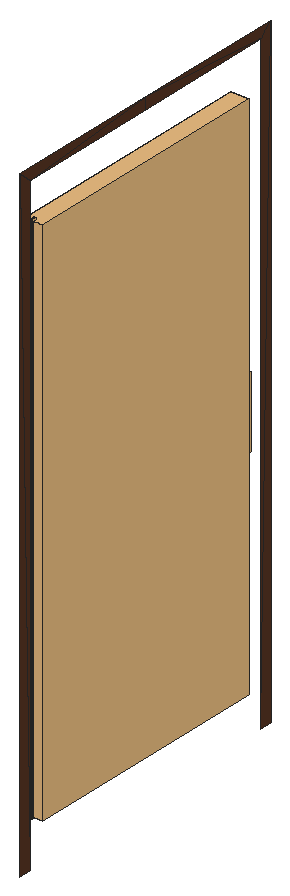
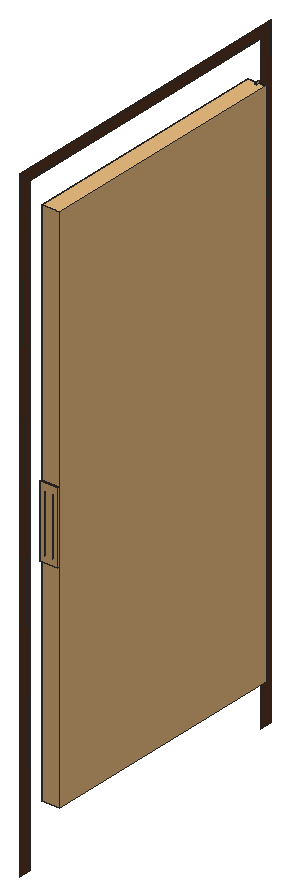
# SketchUp Ruby script. Lengths in inches.
U = 1.inch
M = Sketchup.active_model
def pt(a) = Geom::Point3d.new(a.map { |v| v * U })
def face(e, loops, mat)
  f = e.add_face(loops[0].map { |a| pt(a) })
  loops[1..].each { |l| e.add_face(l.map { |a| pt(a) }).erase! }
  f.material = f.back_material = mat if mat
  f
end
# faces: each face lists its corners as indices into pts; further lists are holes
def faces(e, pts, list, mat = nil) = list.each { |f| face(e, (f[0].is_a?(Array) ? f : [f]).map { |l| l.map { |i| pts[i] } }, mat) }
# xy, xz, yz: faces in a plane at the given z, y or x. An outline is a flat list of corners, or four numbers for a rectangle; further outlines are holes
def ring(l) = l.size == 4 ? [[l[0], l[1]], [l[2], l[1]], [l[2], l[3]], [l[0], l[3]]] : l.each_slice(2).to_a
def flat(e, list, mat, &to3) = list.each { |f| face(e, (f[0].is_a?(Array) ? f : [f]).map { |l| ring(l).map { |u, v| to3.(u, v) } }, mat) }
def xy(e, z, list, mat = nil) = flat(e, list, mat) { |x, y| [x, y, z] }
def xz(e, y, list, mat = nil) = flat(e, list, mat) { |x, z| [x, y, z] }
def yz(e, x, list, mat = nil) = flat(e, list, mat) { |y, z| [x, y, z] }
def lines(e, pts, list) = list.each { |a, b| e.add_line(pt(pts[a]), pt(pts[b])) }
# prism: a flat outline (further loops are holes) pulled along v
def prism(e, loops, v, mat = nil)
  f = face(e, loops, mat); d = Geom::Vector3d.new(v.map { |x| x * U })
  f.pushpull(f.normal.samedirection?(d) ? d.length : -d.length)
end
def box(e, o, s, mat = nil) = prism(e, [[o, [o[0] + s[0], o[1], o[2]], [o[0] + s[0], o[1] + s[1], o[2]], [o[0], o[1] + s[1], o[2]]]], [0, 0, s[2]], mat)
def at(x, y, z, deg = 0) = Geom::Transformation.translation(pt([x, y, z])) * Geom::Transformation.rotation(ORIGIN, Z_AXIS, deg.degrees)
def axes(o, x, y, z) = Geom::Transformation.new([*x, 0, *y, 0, *z, 0, *pt(o).to_a, 1])
def part(name) = M.definitions.add(name)
# library, detail: a bought-in or finely detailed component or shape, given as its bounding box
def library(name, o, s) = part(name).tap { |d| box(d.entities, o, s) }
def detail(e, o, s) = box(e.add_group.entities, o, s)
def put(e, d, t, mat = nil) = e.add_instance(d, t).tap { |i| i.material = mat if mat }
def group(e, t, mat = nil) = e.add_group.tap { |g| g.transformation = t; g.material = mat if mat }.entities
root = M.entities
M.materials.add("Material \#0").color = [86, 53, 35]
M.materials.add("Material \#1").color = [140, 140, 140]
c1 = library("3DGeom~9_Defintion",[456.52,-471.89,-18.89],[5.57,1000,5.49])
c2 = library("3DGeom~7_Defintion",[455.56,-471.94,-18.85],[5.55,1000,5.48])
c3 = part("3DGeom~8_Defintion")
xz(c3.entities,-471.94,[[458.125,-17.29,459.53,-16.11,457.73,-17.15],[458.125,-17.29,458.54,-17.29,459.53,-16.11],[458.54,-17.29,458.93,-17.15,459.53,-16.11],[457.73,-17.15,459.53,-16.11,457.42,-16.88],[458.93,-17.15,459.25,-16.88,459.53,-16.11],
  [457.42,-16.88,459.53,-16.11,457.21,-16.52],[459.25,-16.88,459.46,-16.52,459.53,-16.11],[457.21,-16.52,459.53,-16.11,457.14,-16.11],[457.14,-16.11,459.53,-16.11,457.21,-15.7],[459.53,-16.11,457.42,-15.34,457.21,-15.7],
  [459.53,-16.11,457.73,-15.07,457.42,-15.34],[459.53,-16.11,458.125,-14.93,457.73,-15.07],[459.53,-16.11,458.54,-14.93,458.125,-14.93],[459.53,-16.11,458.93,-15.07,458.54,-14.93],[459.53,-16.11,459.25,-15.34,458.93,-15.07],
  [459.53,-16.11,459.46,-15.7,459.25,-15.34]],"Material \#1")
xz(c3.entities,-416.39,[[458.125,-17.29,457.73,-17.15,459.53,-16.11],[458.125,-17.29,459.53,-16.11,458.54,-17.29],[458.54,-17.29,459.53,-16.11,458.93,-17.15],[457.73,-17.15,457.42,-16.88,459.53,-16.11],[458.93,-17.15,459.53,-16.11,459.25,-16.88],
  [457.42,-16.88,457.21,-16.52,459.53,-16.11],[459.25,-16.88,459.53,-16.11,459.46,-16.52],[457.21,-16.52,457.14,-16.11,459.53,-16.11],[457.14,-16.11,457.21,-15.7,459.53,-16.11],[459.53,-16.11,457.21,-15.7,457.42,-15.34],
  [459.53,-16.11,457.42,-15.34,457.73,-15.07],[459.53,-16.11,457.73,-15.07,458.125,-14.93],[459.53,-16.11,458.125,-14.93,458.54,-14.93],[459.53,-16.11,458.54,-14.93,458.93,-15.07],[459.53,-16.11,458.93,-15.07,459.25,-15.34],
  [459.53,-16.11,459.25,-15.34,459.46,-15.7]],"Material \#1")
xz(c3.entities,-27.5,[[458.125,-17.29,459.53,-16.11,457.73,-17.15],[458.125,-17.29,458.54,-17.29,459.53,-16.11],[458.54,-17.29,458.93,-17.15,459.53,-16.11],[457.73,-17.15,459.53,-16.11,457.42,-16.88],[458.93,-17.15,459.25,-16.88,459.53,-16.11],
  [457.42,-16.88,459.53,-16.11,457.21,-16.52],[459.25,-16.88,459.46,-16.52,459.53,-16.11],[457.21,-16.52,459.53,-16.11,457.14,-16.11],[457.14,-16.11,459.53,-16.11,457.21,-15.7],[459.53,-16.11,457.42,-15.34,457.21,-15.7],
  [459.53,-16.11,457.73,-15.07,457.42,-15.34],[459.53,-16.11,458.125,-14.93,457.73,-15.07],[459.53,-16.11,458.54,-14.93,458.125,-14.93],[459.53,-16.11,458.93,-15.07,458.54,-14.93],[459.53,-16.11,459.25,-15.34,458.93,-15.07],
  [459.53,-16.11,459.46,-15.7,459.25,-15.34]],"Material \#1")
xz(c3.entities,28.06,[[458.125,-17.29,457.73,-17.15,459.53,-16.11],[458.125,-17.29,459.53,-16.11,458.54,-17.29],[458.54,-17.29,459.53,-16.11,458.93,-17.15],[457.73,-17.15,457.42,-16.88,459.53,-16.11],[458.93,-17.15,459.53,-16.11,459.25,-16.88],
  [457.42,-16.88,457.21,-16.52,459.53,-16.11],[459.25,-16.88,459.53,-16.11,459.46,-16.52],[457.21,-16.52,457.14,-16.11,459.53,-16.11],[457.14,-16.11,457.21,-15.7,459.53,-16.11],[459.53,-16.11,457.21,-15.7,457.42,-15.34],
  [459.53,-16.11,457.42,-15.34,457.73,-15.07],[459.53,-16.11,457.73,-15.07,458.125,-14.93],[459.53,-16.11,458.125,-14.93,458.54,-14.93],[459.53,-16.11,458.54,-14.93,458.93,-15.07],[459.53,-16.11,458.93,-15.07,459.25,-15.34],
  [459.53,-16.11,459.25,-15.34,459.46,-15.7]],"Material \#1")
xz(c3.entities,472.5,[[458.125,-17.29,459.53,-16.11,457.73,-17.15],[458.125,-17.29,458.54,-17.29,459.53,-16.11],[458.54,-17.29,458.93,-17.15,459.53,-16.11],[457.73,-17.15,459.53,-16.11,457.42,-16.88],[458.93,-17.15,459.25,-16.88,459.53,-16.11],
  [457.42,-16.88,459.53,-16.11,457.21,-16.52],[459.25,-16.88,459.46,-16.52,459.53,-16.11],[457.21,-16.52,459.53,-16.11,457.14,-16.11],[457.14,-16.11,459.53,-16.11,457.21,-15.7],[459.53,-16.11,457.42,-15.34,457.21,-15.7],
  [459.53,-16.11,457.73,-15.07,457.42,-15.34],[459.53,-16.11,458.125,-14.93,457.73,-15.07],[459.53,-16.11,458.54,-14.93,458.125,-14.93],[459.53,-16.11,458.93,-15.07,458.54,-14.93],[459.53,-16.11,459.25,-15.34,458.93,-15.07],
  [459.53,-16.11,459.46,-15.7,459.25,-15.34]],"Material \#1")
xz(c3.entities,528.06,[[458.125,-17.29,457.73,-17.15,459.53,-16.11],[458.125,-17.29,459.53,-16.11,458.54,-17.29],[458.54,-17.29,459.53,-16.11,458.93,-17.15],[457.73,-17.15,457.42,-16.88,459.53,-16.11],[458.93,-17.15,459.53,-16.11,459.25,-16.88],
  [457.42,-16.88,457.21,-16.52,459.53,-16.11],[459.25,-16.88,459.53,-16.11,459.46,-16.52],[457.21,-16.52,457.14,-16.11,459.53,-16.11],[457.14,-16.11,457.21,-15.7,459.53,-16.11],[459.53,-16.11,457.21,-15.7,457.42,-15.34],
  [459.53,-16.11,457.42,-15.34,457.73,-15.07],[459.53,-16.11,457.73,-15.07,458.125,-14.93],[459.53,-16.11,458.125,-14.93,458.54,-14.93],[459.53,-16.11,458.54,-14.93,458.93,-15.07],[459.53,-16.11,458.93,-15.07,459.25,-15.34],
  [459.53,-16.11,459.25,-15.34,459.46,-15.7]],"Material \#1")
c4 = part("3DGeom~21_Defintion")
xy(c4.entities,73.08,[[-976.3,-241.71,23.7,-241.71,-976.3,-223.46],[23.7,-241.71,5.45,-223.46,-976.3,-223.46],[23.7,-241.71,23.7,0,5.45,-223.46],[5.45,-223.46,23.7,0,5.45,0],[23.7,0,23.7,241.71,5.45,223.46],
  [5.45,0,23.7,0,5.45,223.46],[-976.3,223.46,23.7,241.71,-976.3,241.71],[-976.3,223.46,5.45,223.46,23.7,241.71]],"Material \#0")
c5 = library("3DGeom~6_Defintion",[-5.59,-471.8,-48.03],[468.87,1000,73.72])
c6 = library("3DGeom~3_Defintion",[-83.33,-500,-350],[620.1,1000,533.33])
c7 = library("3DGeom~4_Defintion",[-18.02,-499.97,-221.16],[36.04,1000,262.12])
c8 = part("3DGeom~5_Defintion")
xy(c8.entities,-225.24,[[-0.79,-499.98,-2.33,-499.64,7.45,-496.14],[-0.79,-499.98,7.45,-496.14,1.58,-499.88],[1.58,-499.88,7.45,-496.14,3.84,-499.16],[-2.33,-499.64,7.4,-485.75,7.45,-496.14],[3.84,-499.16,7.45,-496.14,5.85,-497.89],
  [7.45,-496.14,7.4,-485.75,8.24,-487.08],[7.45,-496.14,8.24,-487.08,8.96,-489.34],[7.45,-496.14,8.96,-489.34,9.0625,-491.71],[7.45,-496.14,9.0625,-491.71,8.55,-494.03],[-7.4,-496.08,-8.24,-494.76,2.32,-482.2],
  [-8.24,-494.76,-8.96,-492.5,2.32,-482.2],[-8.96,-492.5,-9.0625,-490.125,2.32,-482.2],[-9.0625,-490.125,-8.55,-487.81,2.32,-482.2],[-8.55,-487.81,-7.45,-485.7,2.32,-482.2],[-7.45,-485.7,-5.85,-483.95,2.32,-482.2],
  [-5.85,-483.95,-3.84,-482.68,2.32,-482.2],[-3.84,-482.68,-1.58,-481.96,2.32,-482.2],[2.32,-482.2,-1.58,-481.96,0.79,-481.86],[0,481.82,-2.35,482.13,-6.92,496.71],[0,481.82,-6.92,496.71,1.55,482.04],
  [-2.35,482.13,-4.55,483.04,-6.92,496.71],[-4.55,483.04,-6.43,484.49,-6.92,496.71],[-6.43,484.49,-7.88,486.37,-6.92,496.71],[6.92,485.12,-1.55,499.8125,7.88,495.47],[6.92,485.12,7.88,495.47,7.88,486.37],
  [-7.88,486.37,-8.79,488.57,-6.92,496.71],[7.88,486.37,7.88,495.47,8.79,488.57],[-8.79,488.57,-9.1,490.92,-6.92,496.71],[8.79,488.57,7.88,495.47,9.1,490.92],[-9.1,490.92,-8.79,493.28,-6.92,496.71],
  [9.1,490.92,7.88,495.47,8.79,493.28],[-8.79,493.28,-7.88,495.47,-6.92,496.71],[7.88,495.47,-1.55,499.8125,0,500.02],[7.88,495.47,0,500.02,2.35,499.71],[7.88,495.47,2.35,499.71,4.55,498.8],
  [7.88,495.47,4.55,498.8,6.43,497.35]],"Material \#1")
xy(c8.entities,-221.57,[[-2.33,-499.64,-5.22,-498.37,7.4,-485.75],[-5.22,-498.37,-7.4,-496.08,5.22,-483.47],[-5.22,-498.37,5.22,-483.47,7.4,-485.75],[-7.4,-496.08,2.32,-482.2,5.22,-483.47],[1.55,482.04,-6.92,496.71,-4.55,498.8],
  [1.55,482.04,-4.55,498.8,4.55,483.04],[4.55,483.04,-4.55,498.8,-1.55,499.8125],[4.55,483.04,-1.55,499.8125,6.92,485.12]],"Material \#1")
xy(c8.entities,38.05,[[-2.33,-499.64,7.4,-485.75,-5.22,-498.37],[-5.22,-498.37,5.22,-483.47,-7.4,-496.08],[-5.22,-498.37,7.4,-485.75,5.22,-483.47],[-7.4,-496.08,5.22,-483.47,2.32,-482.2],[1.55,482.04,-4.55,498.8,-6.92,496.71],
  [1.55,482.04,4.55,483.04,-4.55,498.8],[4.55,483.04,-1.55,499.8125,-4.55,498.8],[4.55,483.04,6.92,485.12,-1.55,499.8125]],"Material \#1")
xy(c8.entities,41.72,[[-0.79,-499.98,7.45,-496.14,-2.33,-499.64],[-0.79,-499.98,1.58,-499.88,7.45,-496.14],[1.58,-499.88,3.84,-499.16,7.45,-496.14],[-2.33,-499.64,7.45,-496.14,7.4,-485.75],[3.84,-499.16,5.85,-497.89,7.45,-496.14],
  [7.45,-496.14,8.24,-487.08,7.4,-485.75],[7.45,-496.14,8.55,-494.03,9.0625,-491.71],[7.45,-496.14,8.96,-489.34,8.24,-487.08],[7.45,-496.14,9.0625,-491.71,8.96,-489.34],[-7.4,-496.08,2.32,-482.2,-8.24,-494.76],
  [-8.24,-494.76,2.32,-482.2,-8.96,-492.5],[-8.96,-492.5,2.32,-482.2,-9.0625,-490.125],[-9.0625,-490.125,2.32,-482.2,-8.55,-487.81],[-8.55,-487.81,2.32,-482.2,-7.45,-485.7],[-7.45,-485.7,2.32,-482.2,-5.85,-483.95],
  [-5.85,-483.95,2.32,-482.2,-3.84,-482.68],[-3.84,-482.68,2.32,-482.2,-1.58,-481.96],[2.32,-482.2,0.79,-481.86,-1.58,-481.96],[0,481.82,-6.92,496.71,-2.35,482.13],[0,481.82,1.55,482.04,-6.92,496.71],
  [-2.35,482.13,-6.92,496.71,-4.55,483.04],[-4.55,483.04,-6.92,496.71,-6.43,484.49],[-6.43,484.49,-6.92,496.71,-7.88,486.37],[6.92,485.12,7.88,495.47,-1.55,499.8125],[6.92,485.12,7.88,486.37,7.88,495.47],
  [-7.88,486.37,-6.92,496.71,-8.79,488.57],[7.88,486.37,8.79,488.57,7.88,495.47],[-8.79,488.57,-6.92,496.71,-9.1,490.92],[8.79,488.57,9.1,490.92,7.88,495.47],[-9.1,490.92,-6.92,496.71,-8.79,493.28],
  [9.1,490.92,8.79,493.28,7.88,495.47],[-8.79,493.28,-6.92,496.71,-7.88,495.47],[7.88,495.47,0,500.02,-1.55,499.8125],[7.88,495.47,2.35,499.71,0,500.02],[7.88,495.47,4.55,498.8,2.35,499.71],
  [7.88,495.47,6.43,497.35,4.55,498.8]],"Material \#1")
xy(root,7.66,[[363.16,355.99,363.12,356,363.12,356.03],[363.16,355.99,363.12,356.03,363.16,356.01],[363.16,355.99,363.16,356.01,363.2,356],[363.12,356,363.08,356.05,363.09,356.07],[363.12,356,363.09,356.07,363.12,356.03],
  [363.2,356,363.16,356.01,363.19,356.03],[363.2,356,363.19,356.03,363.23,356.05],[363.19,356.03,363.22,356.07,363.23,356.05],[363.08,356.05,363.06,356.12,363.07,356.13],[363.08,356.05,363.07,356.13,363.09,356.07],
  [363.23,356.05,363.22,356.07,363.26,356.12],[363.22,356.07,363.25,356.13,363.26,356.12],[363.06,356.12,363.04,356.2,363.06,356.2],[363.06,356.12,363.06,356.2,363.07,356.13],[363.26,356.12,363.25,356.13,363.27,356.2],
  [363.25,356.13,363.26,356.2,363.27,356.2],[363.04,356.2,363.04,356.29,363.06,356.28],[363.04,356.2,363.06,356.28,363.06,356.2],[363.26,356.2,363.26,356.28,363.27,356.29],[363.26,356.2,363.27,356.29,363.27,356.2],
  [363.06,356.28,363.04,356.29,363.07,356.36],[363.26,356.28,363.25,356.36,363.26,356.37],[363.26,356.28,363.26,356.37,363.27,356.29],[363.04,356.29,363.06,356.37,363.07,356.36],[363.07,356.36,363.06,356.37,363.09,356.42],
  [363.25,356.36,363.22,356.42,363.23,356.4375],[363.25,356.36,363.23,356.4375,363.26,356.37],[363.06,356.37,363.08,356.4375,363.09,356.42],[363.09,356.42,363.08,356.4375,363.12,356.46],[363.22,356.42,363.19,356.46,363.2,356.48],
  [363.22,356.42,363.2,356.48,363.23,356.4375],[363.08,356.4375,363.12,356.48,363.12,356.46],[363.12,356.46,363.12,356.48,363.16,356.47],[363.19,356.46,363.16,356.47,363.16,356.49],[363.19,356.46,363.16,356.49,363.2,356.48],
  [363.16,356.47,363.12,356.48,363.16,356.49]],"Material \#1")
xy(root,7.68,[[363.16,355.99,363.16,356.01,363.12,356],[363.16,355.99,363.19,356.03,363.16,356.01],[363.16,355.99,363.2,356,363.19,356.03],[363.12,356,363.12,356.03,363.08,356.05],[363.12,356,363.16,356.01,363.12,356.03],
  [363.2,356,363.22,356.07,363.19,356.03],[363.2,356,363.23,356.05,363.22,356.07],[363.12,356.03,363.09,356.07,363.08,356.05],[363.08,356.05,363.09,356.07,363.06,356.12],[363.23,356.05,363.25,356.13,363.22,356.07],
  [363.23,356.05,363.26,356.12,363.25,356.13],[363.09,356.07,363.07,356.13,363.06,356.12],[363.06,356.12,363.07,356.13,363.04,356.2],[363.26,356.12,363.26,356.2,363.25,356.13],[363.26,356.12,363.27,356.2,363.26,356.2],
  [363.07,356.13,363.06,356.2,363.04,356.2],[363.04,356.2,363.06,356.2,363.04,356.29],[363.06,356.2,363.06,356.28,363.04,356.29],[363.26,356.2,363.27,356.2,363.26,356.28],[363.27,356.2,363.27,356.29,363.26,356.28],
  [363.06,356.28,363.06,356.37,363.04,356.29],[363.06,356.28,363.07,356.36,363.06,356.37],[363.26,356.28,363.27,356.29,363.25,356.36],[363.27,356.29,363.26,356.37,363.25,356.36],[363.07,356.36,363.08,356.4375,363.06,356.37],
  [363.07,356.36,363.09,356.42,363.08,356.4375],[363.25,356.36,363.26,356.37,363.22,356.42],[363.26,356.37,363.23,356.4375,363.22,356.42],[363.09,356.42,363.12,356.48,363.08,356.4375],[363.09,356.42,363.12,356.46,363.12,356.48],
  [363.22,356.42,363.23,356.4375,363.19,356.46],[363.23,356.4375,363.2,356.48,363.19,356.46],[363.12,356.46,363.16,356.47,363.16,356.49],[363.12,356.46,363.16,356.49,363.12,356.48],[363.19,356.46,363.2,356.48,363.16,356.47],
  [363.16,356.47,363.2,356.48,363.16,356.49]],"Material \#1")
xy(root,12.1,[[363.16,355.99,363.12,356,363.16,356.01],[363.16,355.99,363.16,356.01,363.19,356.03],[363.16,355.99,363.19,356.03,363.2,356],[363.12,356,363.08,356.05,363.12,356.03],[363.12,356,363.12,356.03,363.16,356.01],
  [363.2,356,363.19,356.03,363.22,356.07],[363.2,356,363.22,356.07,363.23,356.05],[363.12,356.03,363.08,356.05,363.09,356.07],[363.08,356.05,363.06,356.12,363.09,356.07],[363.23,356.05,363.22,356.07,363.25,356.13],
  [363.23,356.05,363.25,356.13,363.26,356.12],[363.09,356.07,363.06,356.12,363.07,356.13],[363.06,356.12,363.04,356.2,363.07,356.13],[363.26,356.12,363.25,356.13,363.26,356.2],[363.26,356.12,363.26,356.2,363.27,356.2],
  [363.07,356.13,363.04,356.2,363.06,356.2],[363.04,356.2,363.04,356.29,363.06,356.2],[363.06,356.2,363.04,356.29,363.06,356.28],[363.26,356.2,363.26,356.28,363.27,356.2],[363.27,356.2,363.26,356.28,363.27,356.29],
  [363.06,356.28,363.04,356.29,363.06,356.37],[363.06,356.28,363.06,356.37,363.07,356.36],[363.26,356.28,363.25,356.36,363.27,356.29],[363.27,356.29,363.25,356.36,363.26,356.37],[363.07,356.36,363.06,356.37,363.08,356.4375],
  [363.07,356.36,363.08,356.4375,363.09,356.42],[363.25,356.36,363.22,356.42,363.26,356.37],[363.26,356.37,363.22,356.42,363.23,356.4375],[363.09,356.42,363.08,356.4375,363.12,356.48],[363.09,356.42,363.12,356.48,363.12,356.46],
  [363.22,356.42,363.19,356.46,363.23,356.4375],[363.23,356.4375,363.19,356.46,363.2,356.48],[363.12,356.46,363.12,356.48,363.16,356.49],[363.12,356.46,363.16,356.49,363.16,356.47],[363.19,356.46,363.16,356.47,363.2,356.48],
  [363.16,356.47,363.16,356.49,363.2,356.48]],"Material \#1")
xy(root,12.12,[[363.16,355.99,363.12,356.03,363.12,356],[363.16,355.99,363.16,356.01,363.12,356.03],[363.16,355.99,363.2,356,363.16,356.01],[363.12,356,363.09,356.07,363.08,356.05],[363.12,356,363.12,356.03,363.09,356.07],
  [363.2,356,363.19,356.03,363.16,356.01],[363.2,356,363.23,356.05,363.19,356.03],[363.19,356.03,363.23,356.05,363.22,356.07],[363.08,356.05,363.07,356.13,363.06,356.12],[363.08,356.05,363.09,356.07,363.07,356.13],
  [363.23,356.05,363.26,356.12,363.22,356.07],[363.22,356.07,363.26,356.12,363.25,356.13],[363.06,356.12,363.06,356.2,363.04,356.2],[363.06,356.12,363.07,356.13,363.06,356.2],[363.26,356.12,363.27,356.2,363.25,356.13],
  [363.25,356.13,363.27,356.2,363.26,356.2],[363.04,356.2,363.06,356.2,363.06,356.28],[363.04,356.2,363.06,356.28,363.04,356.29],[363.26,356.2,363.27,356.2,363.27,356.29],[363.26,356.2,363.27,356.29,363.26,356.28],
  [363.06,356.28,363.07,356.36,363.04,356.29],[363.26,356.28,363.26,356.37,363.25,356.36],[363.26,356.28,363.27,356.29,363.26,356.37],[363.04,356.29,363.07,356.36,363.06,356.37],[363.07,356.36,363.09,356.42,363.06,356.37],
  [363.25,356.36,363.23,356.4375,363.22,356.42],[363.25,356.36,363.26,356.37,363.23,356.4375],[363.06,356.37,363.09,356.42,363.08,356.4375],[363.09,356.42,363.12,356.46,363.08,356.4375],[363.22,356.42,363.2,356.48,363.19,356.46],
  [363.22,356.42,363.23,356.4375,363.2,356.48],[363.08,356.4375,363.12,356.46,363.12,356.48],[363.12,356.46,363.16,356.47,363.12,356.48],[363.19,356.46,363.16,356.49,363.16,356.47],[363.19,356.46,363.2,356.48,363.16,356.49],
  [363.16,356.47,363.16,356.49,363.12,356.48]],"Material \#1")
yz(root,362.7,[[398.02,43.52,397.86,43.55,397.86,43.53],[398.02,43.52,398.02,43.53,397.86,43.55],[398.02,43.52,398.18,43.53,398.02,43.53],[397.86,43.53,397.71,43.59,397.71,43.57],[397.86,43.53,397.86,43.55,397.71,43.59],
  [398.02,43.53,398.18,43.53,398.17,43.55],[398.18,43.53,398.33,43.57,398.17,43.55],[398.17,43.55,398.33,43.57,398.32,43.59],[397.71,43.57,397.58,43.65,397.57,43.64],[397.71,43.57,397.71,43.59,397.58,43.65],
  [398.33,43.57,398.46,43.64,398.32,43.59],[398.32,43.59,398.46,43.64,398.46,43.65],[397.57,43.64,397.46,43.73,397.45,43.72],[397.57,43.64,397.58,43.65,397.46,43.73],[398.46,43.64,398.59,43.72,398.46,43.65],
  [398.46,43.65,398.59,43.72,398.58,43.73],[397.45,43.72,397.35,43.84,397.34,43.83],[397.45,43.72,397.46,43.73,397.35,43.84],[398.59,43.72,398.69,43.83,398.58,43.73],[398.58,43.73,398.69,43.83,398.68,43.84],
  [397.96,43.75,397.92,43.78,397.91,43.77],[397.96,43.75,397.97,43.77,397.92,43.78],[397.96,43.75,398.02,43.75,397.97,43.77],[398.02,43.75,398.02,43.76,397.97,43.77],[398.02,43.75,398.07,43.75,398.02,43.76],
  [398.07,43.75,398.07,43.77,398.02,43.76],[398.07,43.75,398.12,43.77,398.07,43.77],[397.91,43.77,397.875,43.8,397.87,43.79],[397.91,43.77,397.92,43.78,397.875,43.8],[398.07,43.77,398.12,43.77,398.11,43.78],
  [398.12,43.77,398.17,43.79,398.11,43.78],[398.11,43.78,398.17,43.79,398.16,43.8],[397.87,43.79,397.84,43.83,397.83,43.82],[397.87,43.79,397.875,43.8,397.84,43.83],[398.17,43.79,398.21,43.82,398.16,43.8],
  [398.16,43.8,398.21,43.82,398.2,43.83],[397.83,43.82,397.8,43.86,397.79,43.85],[397.83,43.82,397.84,43.83,397.8,43.86],[398.21,43.82,398.24,43.85,398.2,43.83],[397.34,43.83,397.27,43.95,397.25,43.95],
  [397.34,43.83,397.35,43.84,397.27,43.95],[398.2,43.83,398.24,43.85,398.23,43.86],[398.69,43.83,398.78,43.9375,398.68,43.84],[398.68,43.84,398.78,43.9375,398.76,43.95],[397.79,43.85,397.78,43.9,397.76,43.89],
  [397.79,43.85,397.8,43.86,397.78,43.9],[398.24,43.85,398.27,43.89,398.23,43.86],[398.23,43.86,398.27,43.89,398.26,43.9],[397.76,43.89,397.76,43.94,397.74,43.9375],[397.76,43.89,397.78,43.9,397.76,43.94],
  [398.27,43.89,398.29,43.9375,398.26,43.9],[398.26,43.9,398.29,43.9375,398.28,43.94],[397.74,43.9375,397.74,43.99,397.73,43.99],[397.74,43.9375,397.76,43.94,397.74,43.99],[398.29,43.9375,398.31,43.99,398.28,43.94],
  [398.78,43.9375,398.85,44.08,398.76,43.95],[398.28,43.94,398.31,43.99,398.29,43.99],[397.25,43.95,397.2,44.09,397.1875,44.08],[397.25,43.95,397.27,43.95,397.2,44.09],[398.76,43.95,398.85,44.08,398.83,44.09],
  [397.73,43.99,397.74,44.04,397.72,44.04],[397.73,43.99,397.74,43.99,397.74,44.04],[398.29,43.99,398.31,43.99,398.3125,44.03],[398.29,43.99,398.3125,44.03,398.3,44.03],[398.3,44.03,398.31,44.09,398.29,44.08],
  [398.3,44.03,398.3125,44.03,398.31,44.09],[397.72,44.04,397.74,44.04,397.74,44.08],[397.72,44.04,397.74,44.08,397.73,44.09],[397.1875,44.08,397.16,44.23,397.15,44.23],[397.1875,44.08,397.2,44.09,397.16,44.23],
  [397.74,44.08,397.76,44.13,397.73,44.09],[398.29,44.08,398.29,44.14,398.28,44.13],[398.29,44.08,398.31,44.09,398.29,44.14],[398.85,44.08,398.89,44.23,398.83,44.09],[397.73,44.09,397.76,44.13,397.74,44.14],
  [398.83,44.09,398.89,44.23,398.875,44.23],[397.76,44.13,397.78,44.17,397.74,44.14],[398.28,44.13,398.27,44.18,398.26,44.17],[398.28,44.13,398.29,44.14,398.27,44.18],[397.74,44.14,397.78,44.17,397.76,44.18],
  [397.78,44.17,397.8,44.21,397.76,44.18],[398.26,44.17,398.24,44.22,398.23,44.21],[398.26,44.17,398.27,44.18,398.24,44.22],[397.76,44.18,397.8,44.21,397.79,44.22],[397.8,44.21,397.84,44.24,397.79,44.22],
  [398.23,44.21,398.21,44.26,398.2,44.24],[398.23,44.21,398.24,44.22,398.21,44.26],[397.79,44.22,397.84,44.24,397.83,44.26],[397.15,44.23,397.15,44.39,397.13,44.39],[397.15,44.23,397.16,44.23,397.15,44.39],
  [398.875,44.23,398.89,44.23,398.9,44.39],[398.875,44.23,398.9,44.39,398.89,44.39],[397.84,44.24,397.875,44.27,397.83,44.26],[398.2,44.24,398.17,44.28,398.16,44.27],[398.2,44.24,398.21,44.26,398.17,44.28],
  [397.83,44.26,397.875,44.27,397.87,44.28],[397.875,44.27,397.92,44.29,397.87,44.28],[398.16,44.27,398.12,44.3,398.11,44.29],[398.16,44.27,398.17,44.28,398.12,44.3],[397.87,44.28,397.92,44.29,397.91,44.3],
  [397.92,44.29,397.97,44.3,397.91,44.3],[398.11,44.29,398.07,44.32,398.07,44.3],[398.11,44.29,398.12,44.3,398.07,44.32],[397.91,44.3,397.97,44.3,397.96,44.32],[397.97,44.3,398.02,44.31,397.96,44.32],
  [398.07,44.3,398.02,44.32,398.02,44.31],[398.07,44.3,398.07,44.32,398.02,44.32],[398.02,44.31,398.02,44.32,397.96,44.32],[397.13,44.39,397.15,44.39,397.15,52.11],[397.13,44.39,397.15,52.11,397.15,54.24],
  [397.13,44.39,397.15,54.24,397.13,54.24],[398.89,44.39,398.9,44.39,398.9,54.24],[398.89,44.39,398.9,54.24,398.89,54.24]],"Material \#1")
yz(root,364.03,[[398.02,43.52,397.86,43.53,397.86,43.55],[397.86,43.53,397.71,43.57,397.71,43.59],[397.86,43.53,397.71,43.59,397.86,43.55],[397.71,43.57,397.57,43.64,397.58,43.65],[397.71,43.57,397.58,43.65,397.71,43.59],
  [397.57,43.64,397.45,43.72,397.46,43.73],[397.57,43.64,397.46,43.73,397.58,43.65],[397.45,43.72,397.34,43.83,397.35,43.84],[397.45,43.72,397.35,43.84,397.46,43.73],[397.96,43.75,397.92,43.78,397.97,43.77],
  [397.96,43.75,397.97,43.77,398.02,43.75],[398.02,43.75,397.97,43.77,398.02,43.76],[398.17,43.79,398.16,43.8,398.21,43.82],[398.16,43.8,398.2,43.83,398.21,43.82],[398.21,43.82,398.2,43.83,398.24,43.85],
  [397.34,43.83,397.25,43.95,397.27,43.95],[397.34,43.83,397.27,43.95,397.35,43.84],[398.2,43.83,398.23,43.86,398.24,43.85],[397.79,43.85,397.76,43.89,397.78,43.9],[397.76,43.89,397.74,43.9375,397.76,43.94],
  [397.76,43.89,397.76,43.94,397.78,43.9],[397.74,43.9375,397.73,43.99,397.74,43.99],[397.74,43.9375,397.74,43.99,397.76,43.94],[397.25,43.95,397.1875,44.08,397.2,44.09],[397.25,43.95,397.2,44.09,397.27,43.95],
  [397.73,43.99,397.72,44.04,397.74,44.04],[397.73,43.99,397.74,44.04,397.74,43.99],[397.72,44.04,397.73,44.09,397.74,44.08],[397.72,44.04,397.74,44.08,397.74,44.04],[397.1875,44.08,397.15,44.23,397.16,44.23],
  [397.1875,44.08,397.16,44.23,397.2,44.09],[397.74,44.08,397.73,44.09,397.76,44.13],[397.73,44.09,397.74,44.14,397.76,44.13],[397.76,44.13,397.74,44.14,397.78,44.17],[397.74,44.14,397.76,44.18,397.78,44.17],
  [397.78,44.17,397.76,44.18,397.8,44.21],[398.26,44.17,398.23,44.21,398.24,44.22],[397.76,44.18,397.79,44.22,397.8,44.21],[398.23,44.21,398.2,44.24,398.21,44.26],[398.23,44.21,398.21,44.26,398.24,44.22],
  [397.15,44.23,397.13,44.39,397.15,44.39],[397.15,44.23,397.15,44.39,397.16,44.23],[398.2,44.24,398.16,44.27,398.17,44.28],[398.2,44.24,398.17,44.28,398.21,44.26],[397.83,44.26,397.87,44.28,397.875,44.27],
  [397.875,44.27,397.87,44.28,397.92,44.29],[398.16,44.27,398.11,44.29,398.12,44.3],[398.16,44.27,398.12,44.3,398.17,44.28],[397.87,44.28,397.91,44.3,397.92,44.29],[397.92,44.29,397.91,44.3,397.97,44.3],
  [398.11,44.29,398.07,44.3,398.07,44.32],[398.11,44.29,398.07,44.32,398.12,44.3],[397.97,44.3,397.96,44.32,398.02,44.31],[398.07,44.3,398.02,44.31,398.02,44.32],[398.07,44.3,398.02,44.32,398.07,44.32],
  [398.02,44.31,397.96,44.32,398.02,44.32],[397.13,44.39,397.13,54.24,397.15,54.24],[397.13,44.39,397.15,52.11,397.15,44.39],[397.13,44.39,397.15,54.24,397.15,52.11],[398.89,44.39,398.89,54.24,398.9,54.24],
  [398.89,44.39,398.9,54.24,398.9,44.39]],"Material \#1")
p = [[362.7,398.04,43.94],[362.71,398.04,43.94],[362.71,397.94,44.09],[362.7,397.94,44.09],[364.03,398.04,43.94],[364.03,397.94,44.09],
  [364.01,397.94,44.09],[364.01,398.04,43.94],[362.7,398.0625,43.91],[362.72,398.0625,43.91],[364.03,398.0625,43.91],[364.01,398.0625,43.91],
  [362.7,398.12,43.95],[362.72,398.12,43.95],[362.72,398.14,43.92],[362.7,398.14,43.92],[362.72,398.12,43.9],[362.7,398.12,43.9],
  [362.72,398.08,43.88],[362.7,398.08,43.88],[364.03,398.12,43.95],[364.02,398.14,43.92],[364.01,398.14,43.92],[364.01,398.12,43.95],
  [364.02,398.12,43.9],[364.01,398.12,43.9],[364.02,398.08,43.88],[364.01,398.08,43.88],[362.7,397.99,44.13],[362.71,397.99,44.13],
  [362.71,398.1,43.98],[362.7,398.1,43.98],[364.03,397.99,44.13],[364.03,398.1,43.98],[364.01,398.1,43.98],[364.01,397.99,44.13],
  [362.72,397.92,44.12],[362.7,397.92,44.12],[362.72,397.89,44.15],[362.7,397.89,44.15],[364.03,397.92,44.12],[364.01,397.92,44.12],
  [364.02,397.89,44.15],[364.01,397.89,44.15],[362.7,397.97,44.16],[362.72,397.97,44.16],[364.03,397.97,44.16],[364.01,397.97,44.16],
  [362.72,397.92,44.17],[362.7,397.92,44.17],[362.72,397.95,44.1875],[362.7,397.95,44.1875],[364.02,397.92,44.17],[364.01,397.92,44.17],
  [364.02,397.95,44.1875],[364.01,397.95,44.1875]]
faces(root,p,[[0,1,2],[2,3,0],[4,5,6],[6,7,4],[8,9,1],[1,0,8],[10,4,7],[7,11,10],
  [12,13,14],[14,15,12],[15,14,16],[16,17,15],[17,16,18],[18,19,17],[19,18,9],[9,8,19],
  [20,21,22],[22,23,20],[21,24,25],[25,22,21],[24,26,27],[27,25,24],[26,10,11],[11,27,26],
  [28,29,30],[30,31,28],[32,33,34],[34,35,32],[31,30,13],[13,12,31],[33,20,23],[23,34,33],
  [3,2,36],[36,37,3],[37,36,38],[38,39,37],[5,40,41],[41,6,5],[40,42,43],[43,41,40],
  [44,45,29],[29,28,44],[46,32,35],[35,47,46],[39,38,48],[48,49,39],[49,48,50],[50,51,49],
  [51,50,45],[45,44,51],[42,52,53],[53,43,42],[52,54,55],[55,53,52],[54,46,47],[47,55,54]],"Material \#1")
put(root,c1,axes([363.82,398.02,49.3125],[0,-0.09095,0],[0,0,0.08858],[0.04118,0,0]),"Material \#1")
put(root,c2,axes([363.82,398.02,49.3125],[0,-0.09115,0],[0,0,0.08876],[0.04127,0,0]),"Material \#1")
put(root,c3,axes([363.82,398.02,49.3125],[0,-0.09115,0],[0,0,0.08876],[0.04127,0,0]),"Material \#1")
put(root,c4,axes([366.71,379.28,101.58],[0,0,0.10405],[0,-0.10684,0],[-0.04838,0,0]),"Material \#0")
put(root,c5,axes([363.82,398.02,49.3125],[0,-0.09066,0],[0,0,0.08829],[0.04105,0,0]),"Material \#1")
put(root,c6,axes([363.82,398.02,49.3125],[0,-0.01215,0],[0,0,0.01184],[0.0055,0,0]),"Material \#1")
put(root,c7,axes([363.82,398.02,49.3125],[0,-0.01124,0],[0,0,0.01095],[0.00509,0,0]),"Material \#1")
put(root,c8,axes([363.82,398.02,49.3125],[0,-0.01104,0],[0,0,0.01075],[0.005,0,0]),"Material \#1")
